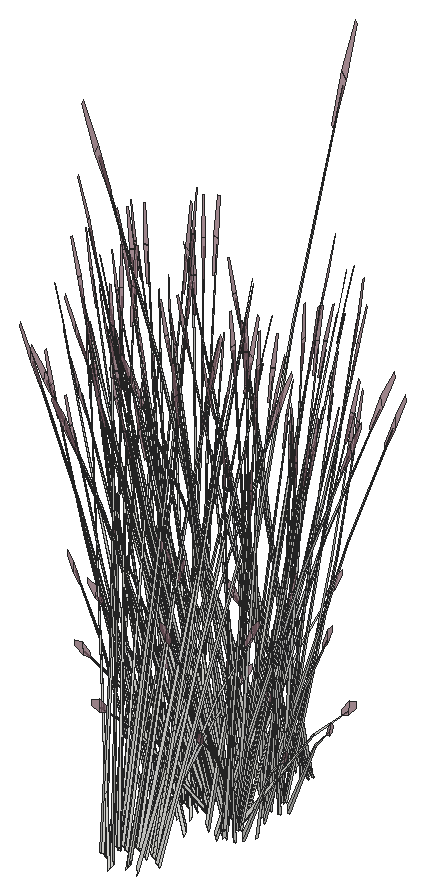
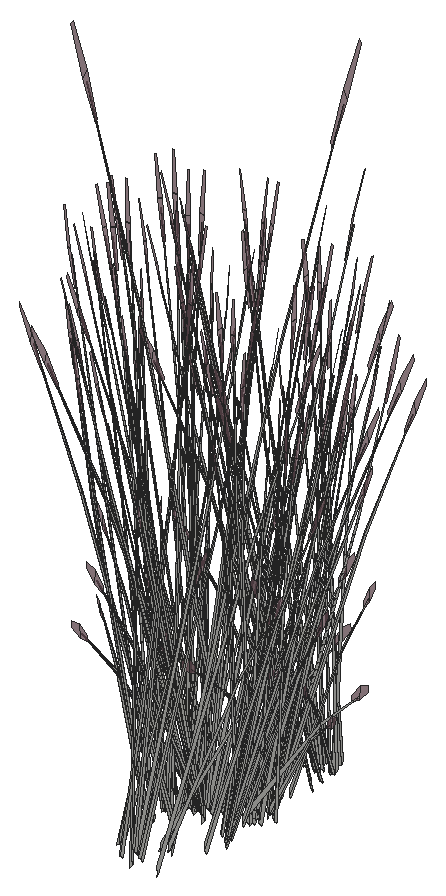
# SketchUp Ruby script. Lengths in inches.
U = 1.inch
M = Sketchup.active_model
def pt(a) = Geom::Point3d.new(a.map { |v| v * U })
def face(e, loops, mat)
  f = e.add_face(loops[0].map { |a| pt(a) })
  loops[1..].each { |l| e.add_face(l.map { |a| pt(a) }).erase! }
  f.material = f.back_material = mat if mat
  f
end
# faces: each face lists its corners as indices into pts; further lists are holes
def faces(e, pts, list, mat = nil) = list.each { |f| face(e, (f[0].is_a?(Array) ? f : [f]).map { |l| l.map { |i| pts[i] } }, mat) }
# xy, xz, yz: faces in a plane at the given z, y or x. An outline is a flat list of corners, or four numbers for a rectangle; further outlines are holes
def ring(l) = l.size == 4 ? [[l[0], l[1]], [l[2], l[1]], [l[2], l[3]], [l[0], l[3]]] : l.each_slice(2).to_a
def flat(e, list, mat, &to3) = list.each { |f| face(e, (f[0].is_a?(Array) ? f : [f]).map { |l| ring(l).map { |u, v| to3.(u, v) } }, mat) }
def xy(e, z, list, mat = nil) = flat(e, list, mat) { |x, y| [x, y, z] }
def xz(e, y, list, mat = nil) = flat(e, list, mat) { |x, z| [x, y, z] }
def yz(e, x, list, mat = nil) = flat(e, list, mat) { |y, z| [x, y, z] }
def lines(e, pts, list) = list.each { |a, b| e.add_line(pt(pts[a]), pt(pts[b])) }
# prism: a flat outline (further loops are holes) pulled along v
def prism(e, loops, v, mat = nil)
  f = face(e, loops, mat); d = Geom::Vector3d.new(v.map { |x| x * U })
  f.pushpull(f.normal.samedirection?(d) ? d.length : -d.length)
end
def box(e, o, s, mat = nil) = prism(e, [[o, [o[0] + s[0], o[1], o[2]], [o[0] + s[0], o[1] + s[1], o[2]], [o[0], o[1] + s[1], o[2]]]], [0, 0, s[2]], mat)
def at(x, y, z, deg = 0) = Geom::Transformation.translation(pt([x, y, z])) * Geom::Transformation.rotation(ORIGIN, Z_AXIS, deg.degrees)
def axes(o, x, y, z) = Geom::Transformation.new([*x, 0, *y, 0, *z, 0, *pt(o).to_a, 1])
def part(name) = M.definitions.add(name)
# library, detail: a bought-in or finely detailed component or shape, given as its bounding box
def library(name, o, s) = part(name).tap { |d| box(d.entities, o, s) }
def detail(e, o, s) = box(e.add_group.entities, o, s)
def put(e, d, t, mat = nil) = e.add_instance(d, t).tap { |i| i.material = mat if mat }
def group(e, t, mat = nil) = e.add_group.tap { |g| g.transformation = t; g.material = mat if mat }.entities
root = M.entities
M.materials.add("LightPink_Translucent").color = [144, 107, 117]
M.materials["LightPink_Translucent"].alpha = 0.75
c1 = part("blade")
p = [[2.15,0.21,22],[0,0.17,0],[0.09,0.45,0],[2.18,0.31,22],[2.29,0.31,22],[0.38,0.45,0],
  [2.48,0.24,33],[2.49,0.24,33],[2.48,0.22,33]]
faces(c1.entities,p,[[0,1,2,3],[4,5,2,3],[6,3,4,7],[8,0,3,6]])
c2 = part("seeds")
p = [[0.3,-0.1,1.38],[-0.01,-0.03,1.59],[-0.01,-0.03,0.03],[0.14,-0.07,-0.07],[0.29,-0.03,3],[0.15,0.01,3.11]]
faces(c2.entities,p,[[0,1,2,3],[1,0,4,5]],"LightPink_Translucent")
c3 = part("blade with seeds")
put(c3.entities,c1,at(0,0,0))
put(c3.entities,c2,axes([2.4,0.25,30.99],[1.5799,-0.05474,1.17369],[-0.12525,1.92788,0.29478],[-0.07173,-0.02425,1.56792]))
put(root,c3,axes([427.33,450.52,154.25],[0.37908,0.26007,-0.10273],[-0.21839,0.37663,-0.57019],[-0.1071,0.13092,0.8664]))
put(root,c3,axes([429.61,451.87,154.25],[0.2442,-0.40372,-0.10273],[0.35364,0.23259,-0.57019],[0.12293,0.11406,0.8664]))
put(root,c3,axes([431.81,455.82,153.98],[-0.05353,-0.00358,1.49853],[-0.22227,-0.38383,-0.1416],[0.08926,-0.1262,0.26519]))
put(root,c3,axes([427.84,450.41,153.27],[0.10236,-0.14492,1.44779],[0.25844,0.39118,0.11706],[-0.17726,0.17814,0.61892]))
put(root,c3,axes([427.52,450.83,153.95],[0.10528,0.43067,-0.43168],[-0.39868,0.07534,-0.33437],[-0.11425,0.11568,0.82598]))
put(root,c3,axes([429.29,452.2,153.98],[0.00121,-0.0571,1.49853],[0.35119,-0.25193,-0.1416],[0.12199,0.08992,0.26519]))
put(root,c3,axes([427.75,451.55,154],[-0.33677,-0.02198,0.05432],[0.00923,-0.33185,0.42765],[-0.03524,0.12712,0.65209]))
put(root,c3,axes([430.98,455.67,153.82],[0.35672,-0.06741,-0.29918],[0.09419,0.38534,0.38624],[0.10222,-0.1035,0.73904]))
put(root,c3,axes([427.85,451.58,154],[-0.29182,-0.32181,0.40553],[0.3099,-0.27755,0.33437],[-0.05383,0.15098,0.83914]))
put(root,c3,axes([429.9,451.67,153.95],[0.40438,-0.11212,-0.43168],[0.07074,0.4246,-0.33437],[0.10862,0.12168,0.82598]))
put(root,c3,axes([427.63,455.02,154],[0.02064,-0.35866,0.05432],[0.3116,0.00983,0.42765],[-0.11936,-0.03753,0.65209]))
put(root,c3,axes([427.51,455.14,153.82],[-0.23317,-0.29531,-0.29918],[0.26625,-0.27955,0.38624],[-0.13527,-0.04253,0.73904]))
put(root,c3,axes([428.2,458.09,153.27],[0.09368,0.15143,1.44779],[-0.43286,0.12749,0.11706],[-0.09783,-0.23774,0.61892]))
put(root,c3,axes([428.91,457.09,153.98],[-0.06268,-0.06613,1.47793],[-0.4183,0.04193,-0.23373],[-0.06676,-0.15817,0.11853]))
put(root,c3,axes([429.7,452.02,154],[-0.18625,0.29962,0.05432],[-0.26523,-0.17444,0.42765],[0.08575,0.09606,0.65209]))
put(root,c3,axes([429.78,451.93,154],[-0.4076,0.10824,0.40553],[-0.07074,-0.4246,0.33437],[0.09586,0.12514,0.83914]))
put(root,c3,axes([427.77,450.76,153.27],[0.0763,-0.16212,1.44779],[0.3201,0.3355,0.11706],[-0.1444,0.2091,0.61892]))
put(root,c3,axes([431.01,455.83,154],[0.28133,0.19836,0.05432],[-0.16379,0.28248,0.42765],[0.0902,-0.09132,0.65209]))
put(root,c3,axes([430.93,455.75,154],[0.10163,0.43409,0.40553],[-0.39868,0.07534,0.33437],[0.1175,-0.10209,0.83914]))
put(root,c3,axes([428.66,452.0625,154],[-0.30197,0.1603,0.05432],[-0.1478,-0.29231,0.42765],[0.02916,0.12885,0.65209]))
put(root,c3,axes([432.01,456.27,153.98],[0.05687,-0.07184,1.47793],[-0.07279,-0.44069,-0.23373],[0.14268,-0.08356,0.11853]))
put(root,c3,axes([427.85,451.68,153.82],[-0.27728,0.24833,-0.29918],[-0.26248,-0.28355,0.38624],[-0.03994,0.14407,0.73904]))
put(root,c3,axes([426.9,451.6,153.98],[-0.01019,0.09334,1.47793],[0.28908,0.3247,-0.23373],[-0.07568,0.15355,0.11853]))
put(root,c3,axes([427.82,451.39,154.56],[0.45039,0.02337,-0.11403],[-0.01231,0.44247,-0.63292],[-0.03129,0.17041,0.9617]))
put(root,c3,axes([428.66,451.89,154.25],[0.40102,-0.2196,-0.10273],[0.19707,0.38974,-0.57019],[0.05291,0.16424,0.8664]))
put(root,c3,axes([430.79,457.9,153.98],[-0.00396,-0.09387,1.47793],[-0.33411,-0.2713,-0.23373],[0.05166,-0.16446,0.11853]))
put(root,c3,axes([429.39,457.88,153.82],[0.12355,-0.36271,-0.29918],[0.36044,0.10579,0.38624],[-0.03305,-0.14603,0.73904]))
put(root,c3,axes([429.66,458.36,153.27],[-0.0763,0.16212,1.44779],[-0.3201,-0.3355,0.11706],[0.1444,-0.2091,0.61892]))
put(root,c3,axes([430.7,457.5625,153.98],[-0.04162,0.03603,1.49853],[-0.40776,-0.12155,-0.1416],[-0.01476,-0.15722,0.26519]))
put(root,c3,axes([427.2,454.55,153.98],[0.03038,0.04707,1.49853],[-0.14646,0.42312,-0.1416],[-0.14833,0.00306,0.26519]))
put(root,c3,axes([429.21,458.13,153.95],[-0.40284,-0.11824,-0.43168],[0.13808,-0.40538,-0.33437],[-0.03694,-0.16321,0.82598]))
put(root,c3,axes([427.625,455.43,153.95],[-0.29757,0.31243,-0.43168],[-0.2606,-0.33005,-0.33437],[-0.15119,-0.04754,0.82598]))
put(root,c3,axes([428.13,451.56,154.23],[0.29336,0.31691,-0.47917],[-0.3099,0.27755,-0.37115],[-0.04464,0.16102,0.91684]))
put(root,c3,axes([430.08,458.4375,153.95],[-0.29336,-0.31691,-0.43168],[0.3099,-0.27755,-0.33437],[0.04464,-0.16102,0.82598]))
put(root,c3,axes([429,451.87,153.95],[0.40284,0.11824,-0.43168],[-0.13808,0.40538,-0.33437],[0.03694,0.16321,0.82598]))
put(root,c3,axes([429.23,451.03,153.27],[-0.09368,-0.15143,1.44779],[0.43286,-0.12749,0.11706],[0.09783,0.23774,0.61892]))
put(root,c3,axes([428.49,456.875,153.98],[-0.00765,0.05653,1.49853],[-0.37706,0.20517,-0.1416],[-0.11096,-0.10488,0.26519]))
put(root,c3,axes([427.78,455.1,154.25],[-0.02194,0.47967,-0.10273],[-0.41546,-0.01311,-0.57019],[-0.16001,-0.03332,0.8664]))
put(root,c3,axes([428.82,452.12,153.82],[-0.12355,0.36271,-0.29918],[-0.36044,-0.10579,0.38624],[0.03305,0.14603,0.73904]))
put(root,c3,axes([430.89,456.94,154.25],[-0.20619,-0.42709,-0.10273],[0.36595,-0.20988,-0.57019],[0.15422,-0.05635,0.8664]))
put(root,c3,axes([430.87,456.58,153.95],[0.11102,-0.42903,-0.43168],[0.38064,0.14706,-0.33437],[0.15325,-0.03934,0.82598]))
put(root,c3,axes([427.25,455.76,153.27],[0.16998,-0.01068,1.44779],[-0.11276,0.46299,0.11706],[-0.24224,-0.02864,0.61892]))
put(root,c3,axes([429.43,457.97,154],[0.4038,0.12331,0.40553],[-0.13808,0.40538,0.33437],[-0.02427,-0.15942,0.83914]))
put(root,c3,axes([429.55,458.11,154.25],[-0.40102,0.2196,-0.10273],[-0.19707,-0.38974,-0.57019],[-0.05291,-0.16424,0.8664]))
put(root,c3,axes([428.04,451.41,154.51],[-0.01066,0.43628,-0.66621],[-0.44902,-0.0293,0.0804],[-0.04739,0.18483,0.94242]))
put(root,c3,axes([430.38,458.6,154.25],[-0.45039,-0.02337,-0.10273],[0.01231,-0.44247,-0.57019],[0.03129,-0.17041,0.8664]))
put(root,c3,axes([430.35,458.32,153.82],[0.27728,-0.24833,-0.29918],[0.26248,0.28355,0.38624],[0.03994,-0.14407,0.73904]))
put(root,c3,axes([426.87,452.56,153.98],[0.04649,-0.02848,1.49853],[0.38427,0.18941,-0.1416],[-0.00903,0.15771,0.26519]))
put(root,c3,axes([429.54,457.93,154],[0.30197,-0.1603,0.05432],[0.1478,0.29231,0.42765],[-0.02916,-0.12885,0.65209]))
put(root,c3,axes([428.35,458.01,153.82],[-0.06329,-0.37991,-0.29918],[0.36182,-0.10032,0.38624],[-0.09718,-0.10887,0.73904]))
put(root,c3,axes([428.46,451.11,153.27],[-0.01003,-0.18103,1.44779],[0.43473,0.12009,0.11706],[-0.02689,0.25798,0.61892]))
put(root,c3,axes([428.51,457.98,154],[0.18625,-0.29962,0.05432],[0.26523,0.17444,0.42765],[-0.08575,-0.09606,0.65209]))
put(root,c3,axes([428.5625,452.76,153.98],[0.05195,0.07595,1.47793],[0.41921,0.02984,-0.23373],[0.04216,0.1675,0.11853]))
put(root,c3,axes([427.57,458.57,153.27],[0.15222,0.08126,1.44779],[-0.31502,0.34091,0.11706],[-0.19634,-0.15379,0.61892]))
put(root,c3,axes([427.18,456.11,154],[0.11578,-0.43006,0.40553],[0.38064,0.14706,0.33437],[-0.14969,0.02584,0.83914]))
put(root,c3,axes([427.15,456,154],[-0.15051,-0.3216,0.05432],[0.27447,-0.15741,0.42765],[-0.12099,0.03106,0.65209]))
put(root,c3,axes([428.31,458.33,153.95],[-0.40438,0.11212,-0.43168],[-0.07074,-0.4246,-0.33437],[-0.10862,-0.12168,0.82598]))
put(root,c3,axes([430.35,458.42,154],[0.29182,0.32181,0.40553],[-0.3099,0.27755,0.33437],[0.05383,-0.15098,0.83914]))
put(root,c3,axes([428.59,457.95,154.59],[-0.2735,0.45217,-0.11506],[-0.39608,-0.2605,-0.63862],[-0.13768,-0.12775,0.97037]))
put(root,c3,axes([430.46,458.45,154],[0.33677,0.02198,0.05432],[-0.00923,0.33185,0.42765],[0.03524,-0.12712,0.65209]))
put(root,c3,axes([427.89,452.03,152.84],[0.009,-0.24349,1.30391],[0.40497,0.12861,0.18019],[-0.03509,0.2595,0.61571]))
put(root,c3,axes([431.1,456.77,153.82],[0.34057,0.13158,-0.29918],[-0.09933,0.38387,0.38624],[0.13712,-0.0352,0.73904]))
put(root,c3,axes([430.6875,459.17,153.95],[-0.10528,-0.43067,-0.43168],[0.39868,-0.07534,-0.33437],[0.11425,-0.11568,0.82598]))
put(root,c3,axes([427.1,456.16,153.82],[-0.34057,-0.13158,-0.29918],[0.09933,-0.38387,0.38624],[-0.13712,0.0352,0.73904]))
put(root,c3,axes([427.54,457.82,153.98],[-0.08817,-0.00333,1.47793],[-0.28072,0.33293,-0.23373],[-0.14978,-0.06803,0.11853]))
put(root,c3,axes([430.875,459.48,154.25],[-0.37908,-0.26007,-0.10273],[0.21839,-0.37663,-0.57019],[0.1071,-0.13092,0.8664]))
put(root,c3,axes([430.18,456.3,153.27],[-0.16998,0.01068,1.44779],[0.11276,-0.46299,0.11706],[0.24224,0.02864,0.61892]))
put(root,c3,axes([429.31,460.9,152.81],[0.35414,0.19019,1.27785],[-0.34693,0.40974,0.50532],[-0.1554,-0.24285,1.07126]))
put(root,c3,axes([431.05,456.93,154],[0.15051,0.3216,0.05432],[-0.27447,0.15741,0.42765],[0.12099,-0.03106,0.65209]))
put(root,c3,axes([431.03,456.82,154],[-0.11578,0.43006,0.40553],[-0.38064,-0.14706,0.33437],[0.14969,-0.02584,0.83914]))
put(root,c3,axes([431.81,459.36,153.98],[-0.05353,-0.00358,1.49853],[-0.22227,-0.38383,-0.1416],[0.08926,-0.1262,0.26519]))
put(root,c3,axes([428.14,456.1,152.82],[0.11649,-0.06823,1.49584],[0.04017,0.47639,0.11706],[-0.25231,0.06321,0.53462]))
put(root,c3,axes([430.98,459.21,153.82],[0.35672,-0.06741,-0.29918],[0.09419,0.38534,0.38624],[0.10222,-0.1035,0.73904]))
put(root,c3,axes([427.63,458.57,154],[0.02064,-0.35866,0.05432],[0.3116,0.00983,0.42765],[-0.11936,-0.03753,0.65209]))
put(root,c3,axes([427.51,458.68,153.82],[-0.23317,-0.29531,-0.29918],[0.26625,-0.27955,0.38624],[-0.13527,-0.04253,0.73904]))
put(root,c3,axes([431.71,458.21,153.98],[-0.03706,-0.04129,1.49853],[0.08106,-0.44261,-0.1416],[0.14596,-0.02828,0.26519]))
put(root,c3,axes([426.89,456.42,153.98],[-0.06692,0.06124,1.47793],[0.00569,0.44742,-0.23373],[-0.15339,0.05818,0.11853]))
put(root,c3,axes([427.34,456.36,153.95],[-0.11102,0.42903,-0.43168],[-0.38064,-0.14706,-0.33437],[-0.15325,0.03934,0.82598]))
put(root,c3,axes([427.32,455.99,154.25],[0.20619,0.42709,-0.10273],[-0.36595,0.20988,-0.57019],[-0.15422,0.05635,0.8664]))
put(root,c3,axes([431.39,457.84,153.32],[-0.07843,-0.39649,-0.0295],[0.37072,-0.09115,-0.13375],[0.07742,0.02514,0.44114]))
put(root,c3,axes([430.43,457.83,154.25],[0.02194,-0.47967,-0.10273],[0.41546,0.01311,-0.57019],[0.16001,0.03332,0.8664]))
put(root,c3,axes([431.01,459.38,154],[0.28133,0.19836,0.05432],[-0.16379,0.28248,0.42765],[0.0902,-0.09132,0.65209]))
put(root,c3,axes([430.93,459.3,154],[0.10163,0.43409,0.40553],[-0.39868,0.07534,0.33437],[0.1175,-0.10209,0.83914]))
put(root,c3,axes([432.01,459.82,153.98],[0.05687,-0.07184,1.47793],[-0.07279,-0.44069,-0.23373],[0.14268,-0.08356,0.11853]))
put(root,c3,axes([427.2,458.1,153.98],[0.03038,0.04707,1.49853],[-0.14646,0.42312,-0.1416],[-0.14833,0.00306,0.26519]))
put(root,c3,axes([430.79,457.54,153.98],[0.08791,-0.00798,1.47793],[0.24113,-0.36643,-0.23373],[0.15637,0.04837,0.11853]))
put(root,c3,axes([427.27,457.18,154],[-0.10163,-0.43409,0.40553],[0.39868,-0.07534,0.33437],[-0.1175,0.10209,0.83914]))
put(root,c3,axes([427.19,457.1,154],[-0.28133,-0.19836,0.05432],[0.16379,-0.28248,0.42765],[-0.0902,0.09132,0.65209]))
put(root,c3,axes([427.32,456.58,153.27],[0.14219,-0.09977,1.44779],[0.11971,0.461,0.11706],[-0.22323,0.10419,0.61892]))
put(root,c3,axes([427.625,458.98,153.95],[-0.29757,0.31243,-0.43168],[-0.2606,-0.33005,-0.33437],[-0.15119,-0.04754,0.82598]))
put(root,c3,axes([427.78,458.65,154.25],[-0.02194,0.47967,-0.10273],[-0.41546,-0.01311,-0.57019],[-0.16001,-0.03332,0.8664]))
put(root,c3,axes([430.89,460.49,154.25],[-0.20619,-0.42709,-0.10273],[0.36595,-0.20988,-0.57019],[0.15422,-0.05635,0.8664]))
put(root,c3,axes([430.87,460.125,153.95],[0.11102,-0.42903,-0.43168],[0.38064,0.14706,-0.33437],[0.15325,-0.03934,0.82598]))
put(root,c3,axes([427.25,459.31,153.27],[0.16998,-0.01068,1.44779],[-0.11276,0.46299,0.11706],[-0.24224,-0.02864,0.61892]))
put(root,c3,axes([426.14,456.87,153.98],[0.0523,0.01265,1.49853],[0.16179,0.41674,-0.1416],[-0.10706,0.10938,0.26519]))
put(root,c3,axes([430.69,457.8,153.82],[0.23317,0.29531,-0.29918],[-0.26625,0.27955,0.38624],[0.13527,0.04253,0.73904]))
put(root,c3,axes([430.57,457.91,154],[-0.02064,0.35866,0.05432],[-0.3116,-0.00983,0.42765],[0.11936,0.03753,0.65209]))
put(root,c3,axes([427.23,457.27,153.82],[-0.35672,0.06741,-0.29918],[-0.09419,-0.38534,0.38624],[-0.10222,0.1035,0.73904]))
put(root,c3,axes([430.6,457.8,154],[-0.30217,0.31079,0.40553],[-0.2606,-0.33005,0.33437],[0.14177,0.05733,0.83914]))
put(root,c3,axes([428.2,463.5,153.27],[0.09368,0.15143,1.44779],[-0.43286,0.12749,0.11706],[-0.09783,-0.23774,0.61892]))
put(root,c3,axes([427.18,459.66,154],[0.11578,-0.43006,0.40553],[0.38064,0.14706,0.33437],[-0.14969,0.02584,0.83914]))
put(root,c3,axes([428.91,462.49,153.98],[-0.06268,-0.06613,1.47793],[-0.4183,0.04193,-0.23373],[-0.06676,-0.15817,0.11853]))
put(root,c3,axes([427.15,459.55,154],[-0.15051,-0.3216,0.05432],[0.27447,-0.15741,0.42765],[-0.12099,0.03106,0.65209]))
put(root,c3,axes([429.86,457.04,153.27],[-0.15222,-0.08126,1.44779],[0.31502,-0.34091,0.11706],[0.19634,0.15379,0.61892]))
put(root,c3,axes([429.88,455.97,153.78],[-0.35411,-0.24507,1.16821],[0.37391,-0.38156,0.50405],[0.11425,0.22994,1.12919]))
put(root,c3,axes([427.33,457,154.25],[0.37908,0.26007,-0.10273],[-0.21839,0.37663,-0.57019],[-0.1071,0.13092,0.8664]))
put(root,c3,axes([429.61,458.35,154.25],[0.2442,-0.40372,-0.10273],[0.35364,0.23259,-0.57019],[0.12293,0.11406,0.8664]))
put(root,c3,axes([431.1,460.32,153.82],[0.34057,0.13158,-0.29918],[-0.09933,0.38387,0.38624],[0.13712,-0.0352,0.73904]))
put(root,c3,axes([427.84,456.89,153.27],[0.10236,-0.14492,1.44779],[0.25844,0.39118,0.11706],[-0.17726,0.17814,0.61892]))
put(root,c3,axes([427.52,457.3125,153.95],[0.10528,0.43067,-0.43168],[-0.39868,0.07534,-0.33437],[-0.11425,0.11568,0.82598]))
put(root,c3,axes([427.1,459.71,153.82],[-0.34057,-0.13158,-0.29918],[0.09933,-0.38387,0.38624],[-0.13712,0.0352,0.73904]))
put(root,c3,axes([430.79,463.3,153.98],[-0.00396,-0.09387,1.47793],[-0.33411,-0.2713,-0.23373],[0.05166,-0.16446,0.11853]))
put(root,c3,axes([429.39,463.28,153.82],[0.12355,-0.36271,-0.29918],[0.36044,0.10579,0.38624],[-0.03305,-0.14603,0.73904]))
put(root,c3,axes([429.66,463.76,153.27],[-0.0763,0.16212,1.44779],[-0.3201,-0.3355,0.11706],[0.1444,-0.2091,0.61892]))
put(root,c3,axes([430.7,462.97,153.98],[-0.04162,0.03603,1.49853],[-0.40776,-0.12155,-0.1416],[-0.01476,-0.15722,0.26519]))
put(root,c3,axes([429.29,458.6875,153.98],[0.00121,-0.0571,1.49853],[0.35119,-0.25193,-0.1416],[0.12199,0.08992,0.26519]))
put(root,c3,axes([427.75,458.03,154],[-0.33677,-0.02198,0.05432],[0.00923,-0.33185,0.42765],[-0.03524,0.12712,0.65209]))
put(root,c3,axes([427.85,458.0625,154],[-0.29182,-0.32181,0.40553],[0.3099,-0.27755,0.33437],[-0.05383,0.15098,0.83914]))
put(root,c3,axes([429.9,458.15,153.95],[0.40438,-0.11212,-0.43168],[0.07074,0.4246,-0.33437],[0.10862,0.12168,0.82598]))
put(root,c3,axes([430.18,459.84,153.27],[-0.16998,0.01068,1.44779],[0.11276,-0.46299,0.11706],[0.24224,0.02864,0.61892]))
put(root,c3,axes([429.21,463.53,153.95],[-0.40284,-0.11824,-0.43168],[0.13808,-0.40538,-0.33437],[-0.03694,-0.16321,0.82598]))
put(root,c3,axes([430.08,463.84,153.95],[-0.29336,-0.31691,-0.43168],[0.3099,-0.27755,-0.33437],[0.04464,-0.16102,0.82598]))
put(root,c3,axes([431.05,460.48,154],[0.15051,0.3216,0.05432],[-0.27447,0.15741,0.42765],[0.12099,-0.03106,0.65209]))
put(root,c3,axes([431.03,460.37,154],[-0.11578,0.43006,0.40553],[-0.38064,-0.14706,0.33437],[0.14969,-0.02584,0.83914]))
put(root,c3,axes([428.49,462.28,153.98],[-0.00765,0.05653,1.49853],[-0.37706,0.20517,-0.1416],[-0.11096,-0.10488,0.26519]))
put(root,c3,axes([429.7,458.5,154],[-0.18625,0.29962,0.05432],[-0.26523,-0.17444,0.42765],[0.08575,0.09606,0.65209]))
put(root,c3,axes([429.43,463.37,154],[0.4038,0.12331,0.40553],[-0.13808,0.40538,0.33437],[-0.02427,-0.15942,0.83914]))
put(root,c3,axes([429.78,458.42,154],[-0.4076,0.10824,0.40553],[-0.07074,-0.4246,0.33437],[0.09586,0.12514,0.83914]))
put(root,c3,axes([429.55,463.51,154.25],[-0.40102,0.2196,-0.10273],[-0.19707,-0.38974,-0.57019],[-0.05291,-0.16424,0.8664]))
put(root,c3,axes([428.14,459.64,152.82],[0.11649,-0.06823,1.49584],[0.04017,0.47639,0.11706],[-0.25231,0.06321,0.53462]))
